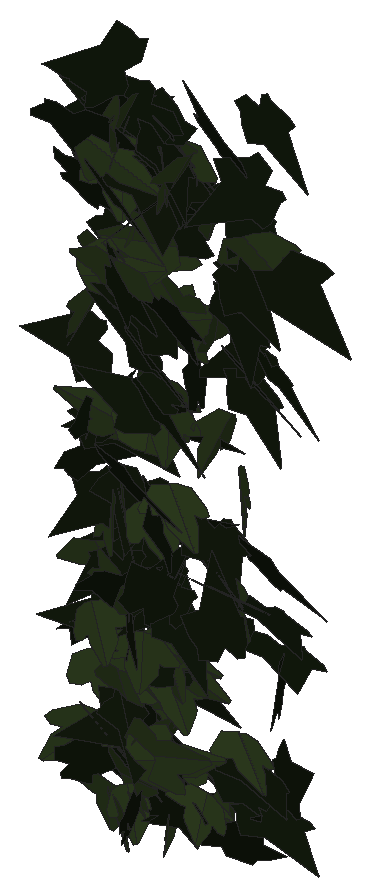
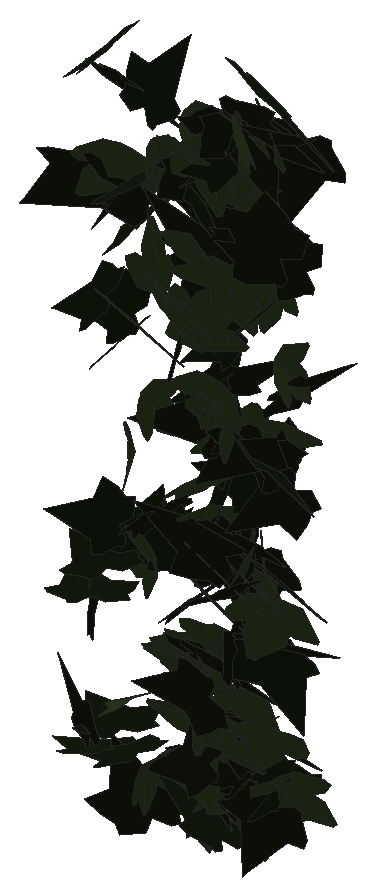
# SketchUp Ruby script. Lengths in inches.
U = 1.inch
M = Sketchup.active_model
def pt(a) = Geom::Point3d.new(a.map { |v| v * U })
def face(e, loops, mat)
  f = e.add_face(loops[0].map { |a| pt(a) })
  loops[1..].each { |l| e.add_face(l.map { |a| pt(a) }).erase! }
  f.material = f.back_material = mat if mat
  f
end
# faces: each face lists its corners as indices into pts; further lists are holes
def faces(e, pts, list, mat = nil) = list.each { |f| face(e, (f[0].is_a?(Array) ? f : [f]).map { |l| l.map { |i| pts[i] } }, mat) }
# xy, xz, yz: faces in a plane at the given z, y or x. An outline is a flat list of corners, or four numbers for a rectangle; further outlines are holes
def ring(l) = l.size == 4 ? [[l[0], l[1]], [l[2], l[1]], [l[2], l[3]], [l[0], l[3]]] : l.each_slice(2).to_a
def flat(e, list, mat, &to3) = list.each { |f| face(e, (f[0].is_a?(Array) ? f : [f]).map { |l| ring(l).map { |u, v| to3.(u, v) } }, mat) }
def xy(e, z, list, mat = nil) = flat(e, list, mat) { |x, y| [x, y, z] }
def xz(e, y, list, mat = nil) = flat(e, list, mat) { |x, z| [x, y, z] }
def yz(e, x, list, mat = nil) = flat(e, list, mat) { |y, z| [x, y, z] }
def lines(e, pts, list) = list.each { |a, b| e.add_line(pt(pts[a]), pt(pts[b])) }
# prism: a flat outline (further loops are holes) pulled along v
def prism(e, loops, v, mat = nil)
  f = face(e, loops, mat); d = Geom::Vector3d.new(v.map { |x| x * U })
  f.pushpull(f.normal.samedirection?(d) ? d.length : -d.length)
end
def box(e, o, s, mat = nil) = prism(e, [[o, [o[0] + s[0], o[1], o[2]], [o[0] + s[0], o[1] + s[1], o[2]], [o[0], o[1] + s[1], o[2]]]], [0, 0, s[2]], mat)
def at(x, y, z, deg = 0) = Geom::Transformation.translation(pt([x, y, z])) * Geom::Transformation.rotation(ORIGIN, Z_AXIS, deg.degrees)
def axes(o, x, y, z) = Geom::Transformation.new([*x, 0, *y, 0, *z, 0, *pt(o).to_a, 1])
def part(name) = M.definitions.add(name)
# library, detail: a bought-in or finely detailed component or shape, given as its bounding box
def library(name, o, s) = part(name).tap { |d| box(d.entities, o, s) }
def detail(e, o, s) = box(e.add_group.entities, o, s)
def put(e, d, t, mat = nil) = e.add_instance(d, t).tap { |i| i.material = mat if mat }
def group(e, t, mat = nil) = e.add_group.tap { |g| g.transformation = t; g.material = mat if mat }.entities
root = M.entities
M.materials.add("1026 AP 7946 SUNNY SIDE UP").color = [254, 231, 186]
M.materials.add("efeu1").color = [18, 25, 13]
M.materials.add("efeu2").color = [43, 57, 29]
c1 = part("ivyleaf_10")
p = [[0,0.5,-0.03],[-0.0625,2.02,-0.43],[-0.19,2.01,-0.46],[-0.54,1.05,-0.29],[-0.52,0.625,-0.18],[-0.83,0.76,-0.28],
  [-1.16,0.64,-0.33],[-1.15,0.33,-0.24],[-0.77,-0.39,0.02],[-0.3,-0.51,0.16],[0.04,-0.48,0.23],[-0.02,2.01,-0.4375],
  [-0.06,2.01,-0.43],[0.04,-0.49,0.23],[0.67,-0.49,0.14],[1.38,0.36,-0.2],[1.375,0.51,-0.24],[0.81,0.65,-0.19],
  [0.62,0.59,-0.15],[0.6,1.09,-0.28],[0.5,1.23,-0.31]]
faces(c1.entities,p,[[0,1,2,3,4,5,6,7,8,9,10],[11,12,0,13,14,15,16,17,18,19,20]],"efeu2")
c2 = part("ivyleaf_9")
p = [[1.54,2.16,1.25],[1.36,2.04,1.19],[-0.21,0.99,0.68],[-0.71,1.11,0.82],[-0.85,0.86,0.67],[-0.8,0.17,0.21],
  [-0.9,-0.01,0.1],[-0.67,-0.16,-0.02],[-0.08,-0.08,-0.05],[-0.03,-0.6,-0.4],[0.65,-0.88,-0.66],[0.83,-0.6,-0.49],
  [1.29,-0.42,-0.43],[1.8125,-0.07,-0.26],[1.21,0.44,0.15]]
faces(c2.entities,p,[[0,1,2,3,4,5,6,7,8,9,10,11,12,13,14]],"efeu1")
put(root,c1,axes([136.93,211.77,280.29],[0.39864,0.12424,-0.25117],[-0.33198,-0.12413,-0.29122],[-0.27527,0.32962,-0.01252]),"1026 AP 7946 SUNNY SIDE UP")
put(root,c2,axes([136.99,212.09,283.83],[-0.49314,0.07212,-0.05929],[0.07158,-0.05806,-0.32851],[-0.12666,-0.31361,0.04519]),"1026 AP 7946 SUNNY SIDE UP")
put(root,c1,axes([136.78,211.9,286.96],[0.07508,-0.29933,0.20921],[0.07253,-0.19986,-0.3132],[0.56563,0.06536,0.01239]),"1026 AP 7946 SUNNY SIDE UP")
put(root,c2,axes([136.35,212.05,288.71],[0.35382,-0.13634,0.24111],[0.27517,-0.16036,-0.26962],[0.32645,0.28295,-0.03405]),"1026 AP 7946 SUNNY SIDE UP")
put(root,c2,axes([136.94,211.81,286.39],[-0.02593,-0.29744,-0.19945],[0.04866,-0.1926,0.30365],[-0.55447,-0.003,0.03598]),"1026 AP 7946 SUNNY SIDE UP")
put(root,c2,axes([136.97,211.34,290.16],[0.48674,0.14403,-0.18455],[-0.23274,-0.10677,-0.35096],[-0.27784,0.34177,-0.02932]),"1026 AP 7946 SUNNY SIDE UP")
put(root,c2,axes([136.93,211.94,280.03],[0.49241,0.07392,-0.1205],[-0.17277,-0.04476,-0.33127],[-0.13316,0.33143,-0.01579]),"1026 AP 7946 SUNNY SIDE UP")
put(root,c2,axes([136.95,211.55,284.83],[-0.02041,0.07372,-0.35573],[-0.11651,0.3377,0.07903],[0.54348,0.07516,0.00358]),"1026 AP 7946 SUNNY SIDE UP")
put(root,c2,axes([137.24,211.61,282.22],[0.0312,0.33207,-0.12146],[-0.07245,-0.11651,-0.34129],[-0.55033,0.03416,0.03805]),"1026 AP 7946 SUNNY SIDE UP")
put(root,c1,axes([137.03,211.86,283.06],[-0.53499,-0.12644,-0.08536],[0.14347,-0.01126,-0.37157],[0.18874,-0.34983,0.04049]),"1026 AP 7946 SUNNY SIDE UP")
put(root,c1,axes([136.92,211.98,281.19],[0.45961,0.15509,0.09905],[0.14745,0.02614,-0.34011],[-0.24529,0.30632,-0.01886]),"1026 AP 7946 SUNNY SIDE UP")
put(root,c2,axes([137.57,211.58,291],[-0.40272,0.31992,0.15659],[-0.18475,0.09785,-0.42057],[-0.5241,-0.28032,0.02793]),"1026 AP 7946 SUNNY SIDE UP")
put(root,c2,axes([137.04,212.34,287.77],[-0.08885,-0.27068,0.21766],[-0.04299,-0.21146,-0.28578],[0.53971,-0.06141,0.01307]),"1026 AP 7946 SUNNY SIDE UP")
put(root,c2,axes([137.48,211.74,285.4375],[-0.32726,0.25952,0.02281],[-0.07406,-0.01151,-0.33979],[-0.40261,-0.20883,0.04396]),"1026 AP 7946 SUNNY SIDE UP")
put(root,c2,axes([137.08,211.49,285.16],[0.0005,-0.04609,0.36122],[0.3436,0.27604,0.03876],[-0.43773,0.21663,0.03084]),"1026 AP 7946 SUNNY SIDE UP")
put(root,c1,axes([137.28,211.58,288.01],[-0.52163,0.16131,0.0163],[-0.04347,-0.0229,-0.37866],[-0.25099,-0.33128,0.0317]),"1026 AP 7946 SUNNY SIDE UP")
put(root,c2,axes([136.96,211.31,279.91],[0.15307,0.07969,0.30415],[0.42767,0.11804,-0.12471],[-0.2183,0.28713,-0.03105]),"1026 AP 7946 SUNNY SIDE UP")
put(root,c1,axes([137.61,211.49,285.51],[0.14265,0.06466,0.33487],[-0.48667,-0.10294,0.10961],[0.18478,-0.32103,0.03016]),"1026 AP 7946 SUNNY SIDE UP")
put(root,c1,axes([137.62,211.36,290.24],[-0.01233,0.08021,0.39313],[-0.49949,0.21928,-0.05299],[-0.3544,-0.31185,0.061]),"1026 AP 7946 SUNNY SIDE UP")
put(root,c2,axes([137.64,211.68,282.27],[-0.37798,0.00609,0.22191],[-0.3256,-0.09571,-0.23586],[0.09364,-0.30824,0.07564]),"1026 AP 7946 SUNNY SIDE UP")
put(root,c1,axes([137.0625,211.93,283.73],[0.20405,-0.09393,0.31687],[0.34377,-0.21827,-0.16469],[0.37198,0.25325,-0.02162]),"1026 AP 7946 SUNNY SIDE UP")
put(root,c2,axes([136.76,212.14,288.83],[0.2823,-0.08921,0.40928],[0.48788,-0.25204,-0.20397],[0.4158,0.3563,-0.03855]),"1026 AP 7946 SUNNY SIDE UP")
put(root,c1,axes([137.25,212.1,284.03],[-0.07396,0.28083,-0.16562],[0.04185,-0.16017,-0.29428],[-0.50835,-0.05405,-0.00013]),"1026 AP 7946 SUNNY SIDE UP")
put(root,c2,axes([137.52,211.74,283.28],[-0.52581,0.06428,-0.12098],[0.16043,-0.08368,-0.34591],[-0.13707,-0.34453,0.05924]),"1026 AP 7946 SUNNY SIDE UP")
put(root,c1,axes([137.71,211.35,282.95],[-0.20558,0.05575,0.30908],[-0.46464,0.05694,-0.14338],[-0.11777,-0.32198,0.02616]),"1026 AP 7946 SUNNY SIDE UP")
put(root,c1,axes([137.41,212.06,289.93],[-0.07296,0.2067,-0.30985],[-0.07696,-0.30514,-0.20923],[-0.5702,0.01473,0.06789]),"1026 AP 7946 SUNNY SIDE UP")
put(root,c1,axes([137.52,211.5,279.56],[-0.4753,0.04032,0.05069],[-0.08344,-0.03005,-0.3121],[-0.05466,-0.30474,0.03565]),"1026 AP 7946 SUNNY SIDE UP")
put(root,c2,axes([137.04,211.82,280.28],[0.33428,-0.25863,0.16353],[0.14298,-0.13249,-0.34543],[0.4565,0.23088,-0.01155]),"1026 AP 7946 SUNNY SIDE UP")
put(root,c2,axes([137.62,211.78,290.4],[0.10188,0.28319,-0.2249],[-0.04468,-0.21872,-0.30006],[-0.56202,0.06872,-0.01691]),"1026 AP 7946 SUNNY SIDE UP")
put(root,c2,axes([137.88,211.78,290.48],[-0.0149,-0.04687,-0.3811],[-0.41566,-0.25977,0.03939],[-0.41294,0.26317,-0.0259]),"1026 AP 7946 SUNNY SIDE UP")
put(root,c1,axes([137.43,211.22,282.47],[0.17588,0.31826,0.00948],[0.01533,0.00441,-0.34741],[-0.50033,0.11201,-0.00731]),"1026 AP 7946 SUNNY SIDE UP")
put(root,c1,axes([137.7,211.3,288.02],[-0.5876,0.01666,0.09381],[-0.14501,-0.03868,-0.3832],[-0.01093,-0.38266,0.04055]),"1026 AP 7946 SUNNY SIDE UP")
put(root,c1,axes([137.57,211.83,290.39],[0.12966,-0.36137,0.10034],[0.01711,-0.09948,-0.38226],[0.5891,0.08243,-0.01098]),"1026 AP 7946 SUNNY SIDE UP")
put(root,c1,axes([137.67,212,287.94],[-0.11616,-0.31092,0.12575],[-0.03937,-0.12132,-0.32991],[0.52476,-0.07793,0.00309]),"1026 AP 7946 SUNNY SIDE UP")
put(root,c1,axes([137.6,211.64,281.3],[-0.52558,0.10178,-0.02684],[0.02429,-0.04026,-0.35849],[-0.16363,-0.33289,0.03299]),"1026 AP 7946 SUNNY SIDE UP")
put(root,c2,axes([137.55,212.1,284.18],[-0.41017,-0.13512,-0.16325],[0.27891,-0.0133,-0.29061],[0.16981,-0.30453,0.08299]),"1026 AP 7946 SUNNY SIDE UP")
put(root,c2,axes([137.36,211.68,285.5],[-0.0797,-0.14271,-0.3437],[0.18445,0.31147,-0.15418],[0.5387,-0.12776,0.00194]),"1026 AP 7946 SUNNY SIDE UP")
put(root,c2,axes([137.95,211.49,280.83],[-0.48105,0.05626,0.10725],[-0.16986,-0.01715,-0.31857],[-0.07486,-0.3226,0.03369]),"1026 AP 7946 SUNNY SIDE UP")
put(root,c2,axes([138.07,211.73,290.01],[-0.09325,0.09619,0.38084],[-0.57632,0.08915,-0.08407],[-0.16621,-0.36308,0.07785]),"1026 AP 7946 SUNNY SIDE UP")
put(root,c1,axes([137.49,211.66,289.4],[0.52881,0.09615,0.04929],[0.08272,-0.01243,-0.35941],[-0.14678,0.33939,-0.02498]),"1026 AP 7946 SUNNY SIDE UP")
put(root,c1,axes([137.98,211.99,280.94],[0.22627,-0.0863,-0.30651],[-0.43366,0.11255,-0.17067],[0.22023,0.31028,-0.02115]),"1026 AP 7946 SUNNY SIDE UP")
put(root,c1,axes([137.35,211.47,289.72],[-0.30172,-0.09486,-0.29096],[0.46756,-0.0538,-0.19019],[0.0103,-0.33673,0.11017]),"1026 AP 7946 SUNNY SIDE UP")
put(root,c2,axes([137.42,211.79,283.93],[0.06748,-0.0427,-0.33349],[0.46238,-0.13631,0.05793],[-0.22231,-0.29648,0.01925]),"1026 AP 7946 SUNNY SIDE UP")
put(root,c2,axes([137.61,211.97,282],[0.04782,0.13868,0.42312],[-0.20909,-0.38806,0.14314],[0.64754,-0.13555,0.01497]),"1026 AP 7946 SUNNY SIDE UP")
put(root,c2,axes([137.37,211.38,289.33],[0.45675,-0.28252,0.02223],[-0.00415,-0.03588,-0.4167],[0.44572,0.28919,-0.02665]),"1026 AP 7946 SUNNY SIDE UP")
put(root,c1,axes([137.68,211.32,279.52],[-0.28001,0.24647,-0.06538],[0.04102,-0.06108,-0.31326],[-0.39864,-0.17941,0.01369]),"1026 AP 7946 SUNNY SIDE UP")
put(root,c1,axes([137.36,211.38,287.79],[0.27127,-0.05329,-0.34809],[0.53275,-0.0229,0.18197],[-0.07044,-0.37842,0.03574]),"1026 AP 7946 SUNNY SIDE UP")
put(root,c1,axes([137.7,211.86,290.13],[-0.43098,-0.1805,-0.13712],[0.26228,-0.02579,-0.32044],[0.23429,-0.30316,0.10649]),"1026 AP 7946 SUNNY SIDE UP")
put(root,c1,axes([138.21,211.63,288.44],[0.20931,-0.06662,-0.35581],[-0.51003,0.11855,-0.15182],[0.21244,0.35027,-0.01393]),"1026 AP 7946 SUNNY SIDE UP")
put(root,c2,axes([137.93,211.17,283.27],[0.24956,0.32164,-0.10605],[-0.05102,-0.10072,-0.36977],[-0.52945,0.16131,-0.01436]),"1026 AP 7946 SUNNY SIDE UP")
put(root,c1,axes([138.09,212.03,289.86],[-0.54056,0.04704,0.1359],[-0.21351,-0.02918,-0.35471],[-0.05232,-0.36697,0.04344]),"1026 AP 7946 SUNNY SIDE UP")
put(root,c2,axes([137.8,211.16,288.08],[0.38523,-0.19837,-0.28642],[-0.33456,0.17723,-0.3237],[0.41825,0.32448,0.00488]),"1026 AP 7946 SUNNY SIDE UP")
put(root,c2,axes([138.03,211.64,286.83],[0.03186,-0.3768,0.00791],[0.01782,0.01044,0.38861],[-0.59242,-0.01995,0.01212]),"1026 AP 7946 SUNNY SIDE UP")
put(root,c2,axes([137.86,212.09,283.14],[-0.23185,-0.28732,0.11258],[-0.01615,-0.11832,-0.33051],[0.48402,-0.14158,0.0429]),"1026 AP 7946 SUNNY SIDE UP")
put(root,c2,axes([137.58,211.66,282.66],[0.01739,-0.1062,-0.42378],[0.61113,-0.16223,0.05304],[-0.2675,-0.37752,0.09363]),"1026 AP 7946 SUNNY SIDE UP")
put(root,c2,axes([138.32,211.87,281.91],[-0.3792,0.12599,0.16898],[-0.24642,0.05144,-0.27899],[-0.21087,-0.28668,0.02215]),"1026 AP 7946 SUNNY SIDE UP")
put(root,c2,axes([138.08,211.86,287.07],[0.03316,-0.36637,-0.07033],[0.00736,-0.06603,0.37767],[-0.58537,-0.02159,0.00077]),"1026 AP 7946 SUNNY SIDE UP")
put(root,c1,axes([137.85,211.45,279.63],[0.19775,0.28098,-0.01252],[0.01181,-0.01841,-0.31689],[-0.44218,0.12517,-0.01407]),"1026 AP 7946 SUNNY SIDE UP")
put(root,c1,axes([137.66,211.59,279.8],[-0.25211,-0.00318,0.30787],[0.44287,-0.11509,0.15373],[0.15725,0.31903,0.06063]),"1026 AP 7946 SUNNY SIDE UP")
put(root,c2,axes([137.86,211.72,280.77],[-0.13229,-0.32043,0.09554],[0.01874,-0.10032,-0.33991],[0.525,-0.07716,0.03621]),"1026 AP 7946 SUNNY SIDE UP")
put(root,c2,axes([137.57,211.48,284.69],[0.32168,-0.19696,0.21194],[0.21293,-0.15713,-0.29303],[0.39542,0.24484,-0.01462]),"1026 AP 7946 SUNNY SIDE UP")
put(root,c2,axes([138.22,211.93,283.5],[-0.46967,0.1199,-0.0451],[0.04815,-0.04261,-0.33058],[-0.19522,-0.29897,0.02697]),"1026 AP 7946 SUNNY SIDE UP")
put(root,c1,axes([138.25,212.03,287.18],[-0.54951,0.01534,-0.17674],[-0.26618,0.04213,0.35919],[0.05075,0.38706,-0.0298]),"1026 AP 7946 SUNNY SIDE UP")
put(root,c2,axes([138.31,211.4,285.92],[-0.10603,0.10099,0.33425],[-0.49992,-0.13404,-0.02592],[0.18614,-0.30245,0.12078]),"1026 AP 7946 SUNNY SIDE UP")
put(root,c1,axes([137.83,212,285.75],[-0.25398,0.11138,-0.28256],[0.23753,-0.2385,-0.19237],[-0.40138,-0.21162,0.06495]),"1026 AP 7946 SUNNY SIDE UP")
put(root,c1,axes([138,211.58,285.34],[0.24112,0.299,-0.17953],[0.08725,0.16877,0.34624],[0.5385,-0.16122,0.02429]),"1026 AP 7946 SUNNY SIDE UP")
put(root,c2,axes([138.05,211.12,279.37],[0.01102,0.03272,0.33814],[0.20251,0.30178,-0.03208],[-0.47719,0.12882,-0.0058]),"1026 AP 7946 SUNNY SIDE UP")
put(root,c2,axes([137.69,212.06,290.05],[0.4629,-0.19329,0.09361],[0.08745,-0.08194,-0.36131],[0.32502,0.29734,-0.03611]),"1026 AP 7946 SUNNY SIDE UP")
put(root,c2,axes([137.71,211.76,280.78],[0.0476,-0.02624,-0.35792],[0.54759,-0.00125,0.03136],[-0.00554,-0.34859,0.02478]),"1026 AP 7946 SUNNY SIDE UP")
put(root,c2,axes([138.52,211.78,281.83],[-0.2706,0.13309,0.25627],[-0.38106,0.07776,-0.21578],[-0.22507,-0.29168,0.05722]),"1026 AP 7946 SUNNY SIDE UP")
put(root,c2,axes([138.29,211.77,289.21],[-0.31059,0.1902,-0.24074],[0.11844,-0.24062,-0.26754],[-0.46009,-0.19034,0.09364]),"1026 AP 7946 SUNNY SIDE UP")
put(root,c1,axes([137.9375,211.88,288.12],[-0.2609,-0.19495,0.27417],[0.21236,0.23299,0.26285],[-0.4748,0.21133,-0.03309]),"1026 AP 7946 SUNNY SIDE UP")
put(root,c2,axes([138.27,211.8125,289.49],[0.14862,0.27194,-0.21457],[-0.06905,-0.20628,-0.29699],[-0.53566,0.10204,-0.02125]),"1026 AP 7946 SUNNY SIDE UP")
put(root,c1,axes([138.02,211.46,282.1],[0.49272,0.03166,0.05162],[0.0831,-0.02936,-0.32272],[-0.04165,0.31594,-0.03328]),"1026 AP 7946 SUNNY SIDE UP")
put(root,c1,axes([138.33,211.68,279.75],[-0.4671,0.13496,-0.11276],[-0.13698,0.07364,0.3352],[0.23729,0.30817,-0.02846]),"1026 AP 7946 SUNNY SIDE UP")
put(root,c1,axes([137.9,211.78,289.24],[0.51442,0.12657,0.1416],[0.22163,0.01256,-0.35934],[-0.1916,0.35435,-0.0355]),"1026 AP 7946 SUNNY SIDE UP")
put(root,c2,axes([137.8125,211.7,280.4],[0.48862,-0.13975,0.07202],[0.0794,-0.05929,-0.34974],[0.2331,0.31312,-0.03182]),"1026 AP 7946 SUNNY SIDE UP")
put(root,c2,axes([138.42,211.79,282.98],[-0.54427,0.13064,-0.09453],[0.11461,-0.06757,-0.37969],[-0.22409,-0.35186,0.0354]),"1026 AP 7946 SUNNY SIDE UP")
put(root,c1,axes([138.12,211.8,286.05],[-0.50622,0.09653,-0.11446],[0.15406,-0.06061,-0.34537],[-0.17358,-0.33532,0.02728]),"1026 AP 7946 SUNNY SIDE UP")
put(root,c1,axes([138.27,211.71,280.78],[-0.06162,-0.34843,0.01596],[0.00282,-0.01778,-0.3613],[0.54855,-0.03905,0.00365]),"1026 AP 7946 SUNNY SIDE UP")
put(root,c1,axes([138.07,211.62,284.11],[0.2288,0.31656,0.07793],[0.07518,0.05918,-0.35808],[-0.50557,0.15206,-0.01798]),"1026 AP 7946 SUNNY SIDE UP")
put(root,c2,axes([137.82,212,283.73],[0.38918,0.15023,-0.1758],[0.20617,0.11328,0.29784],[0.29328,-0.27899,0.0239]),"1026 AP 7946 SUNNY SIDE UP")
put(root,c2,axes([137.96,211.46,286.9],[0.4153,-0.23003,-0.01377],[-0.03277,-0.00559,-0.36039],[0.36071,0.26434,-0.01688]),"1026 AP 7946 SUNNY SIDE UP")
put(root,c2,axes([138.14,211.76,289.54],[-0.37671,-0.22839,-0.19083],[0.2571,0.09313,-0.33798],[0.38276,-0.28733,0.03922]),"1026 AP 7946 SUNNY SIDE UP")
put(root,c2,axes([137.9,211.95,279.29],[0.18214,-0.29811,0.10705],[0.48744,0.12929,0.02646],[-0.09847,0.08862,0.32899]),"1026 AP 7946 SUNNY SIDE UP")
put(root,c1,axes([138.23,211.68,289.4375],[-0.37529,0.26142,0.14992],[0.18781,-0.08537,0.363],[0.43011,0.26538,-0.0277]),"1026 AP 7946 SUNNY SIDE UP")
put(root,c2,axes([138.04,212.01,288.39],[-0.19085,0.1032,0.31474],[0.42594,-0.14333,0.16022],[0.27349,0.29524,-0.02989]),"1026 AP 7946 SUNNY SIDE UP")
put(root,c1,axes([138.38,211.73,279.41],[-0.08232,0.30015,-0.02563],[-0.14322,-0.04148,-0.29797],[-0.45164,-0.04156,0.09916]),"1026 AP 7946 SUNNY SIDE UP")
put(root,c2,axes([138.1,211.93,289.69],[0.05397,-0.33812,0.14326],[0.03661,-0.1393,-0.35082],[0.57485,0.04061,0.00889]),"1026 AP 7946 SUNNY SIDE UP")
put(root,c2,axes([138.02,212.05,280.43],[0.40279,-0.19805,0.10107],[0.10606,-0.07476,-0.33354],[0.33177,0.26434,-0.01607]),"1026 AP 7946 SUNNY SIDE UP")
put(root,c2,axes([137.99,211.74,285.6],[0.40634,-0.01604,0.21777],[0.32979,-0.03017,-0.26656],[0.04952,0.33256,-0.01172]),"1026 AP 7946 SUNNY SIDE UP")
put(root,c2,axes([138.32,211.58,283.96],[-0.10613,-0.02388,0.41954],[-0.08522,-0.40874,-0.03633],[0.63599,-0.05876,0.06514]),"1026 AP 7946 SUNNY SIDE UP")
put(root,c2,axes([138.02,212.07,281.48],[0.10649,-0.01567,-0.34843],[0.50877,0.10427,0.0624],[0.15631,-0.3287,0.03428]),"1026 AP 7946 SUNNY SIDE UP")
put(root,c1,axes([138.29,212,289.72],[0.57583,-0.08475,0.10851],[0.14917,-0.05751,-0.38605],[0.15227,0.37683,-0.03215]),"1026 AP 7946 SUNNY SIDE UP")
put(root,c1,axes([138.29,211.84,281.73],[-0.18868,0.03374,-0.31332],[0.20076,-0.29157,-0.08687],[-0.4376,-0.14831,0.09524]),"1026 AP 7946 SUNNY SIDE UP")
put(root,c1,axes([138.32,211.69,285.8],[0.52327,-0.0806,0.10558],[0.141,-0.06415,-0.35077],[0.14961,0.34239,-0.03868]),"1026 AP 7946 SUNNY SIDE UP")
put(root,c2,axes([138.25,211.72,289.99],[0.08627,-0.34522,0.09461],[0.02919,-0.09202,-0.36062],[0.56175,0.0578,0.00421]),"1026 AP 7946 SUNNY SIDE UP")
put(root,c2,axes([138.18,211.48,286.1],[0.36648,-0.29093,0.01799],[-0.00291,-0.02595,-0.38375],[0.45843,0.23241,-0.01682]),"1026 AP 7946 SUNNY SIDE UP")
put(root,c2,axes([138.76,211.42,279.93],[0.18595,-0.00712,-0.34267],[-0.51563,-0.06185,-0.11912],[-0.08796,0.34752,-0.02612]),"1026 AP 7946 SUNNY SIDE UP")
put(root,c2,axes([138.41,211.08,283.03],[-0.11407,-0.02932,0.38547],[0.3977,0.27797,0.07455],[-0.43637,0.261,-0.03282]),"1026 AP 7946 SUNNY SIDE UP")
put(root,c1,axes([138.17,211.69,282.05],[-0.17709,-0.0173,-0.32255],[0.49267,-0.0167,-0.11529],[-0.01554,-0.33222,0.02063]),"1026 AP 7946 SUNNY SIDE UP")
put(root,c1,axes([138.33,211.7,281.48],[0.43326,0.09107,0.12963],[0.20047,0.01193,-0.29766],[-0.13836,0.30246,-0.02536]),"1026 AP 7946 SUNNY SIDE UP")
put(root,c2,axes([138.47,211.37,287.7],[0.50838,-0.04845,-0.1445],[-0.22448,-0.01223,-0.33539],[0.06216,0.35211,-0.02943]),"1026 AP 7946 SUNNY SIDE UP")
put(root,c1,axes([138.71,211.49,289.92],[0.04285,-0.3592,0.10493],[0.00367,-0.10401,-0.37167],[0.58795,0.02683,-0.00533]),"1026 AP 7946 SUNNY SIDE UP")
put(root,c1,axes([138.46,211.66,284.49],[-0.24768,-0.2937,0.03735],[0.33942,-0.14328,-0.2203],[0.31877,-0.07563,0.26359]),"1026 AP 7946 SUNNY SIDE UP")
put(root,c1,axes([138.26,212.03,287.07],[0.26977,-0.15158,-0.32575],[0.4291,-0.16182,0.23214],[-0.3443,-0.32045,0.03408]),"1026 AP 7946 SUNNY SIDE UP")
put(root,c1,axes([138.32,211.74,279.87],[-0.18682,-0.05004,-0.3372],[0.51673,-0.05803,-0.11418],[-0.06016,-0.34307,0.06639]),"1026 AP 7946 SUNNY SIDE UP")
put(root,c1,axes([138.35,211.79,281.79],[-0.17893,-0.02049,-0.3478],[0.49356,-0.13876,-0.10116],[-0.19761,-0.32802,0.06225]),"1026 AP 7946 SUNNY SIDE UP")
put(root,c1,axes([138.36,211.24,280.52],[-0.30723,0.0151,0.35813],[0.54479,0.04427,0.19894],[-0.04915,0.39624,-0.03353]),"1026 AP 7946 SUNNY SIDE UP")
put(root,c2,axes([138.54,211.66,282.66],[0.10145,-0.34726,-0.04131],[-0.01482,0.03703,-0.36364],[0.54911,0.06516,-0.00218]),"1026 AP 7946 SUNNY SIDE UP")
put(root,c1,axes([138.32,211.27,280.48],[0.15932,-0.01386,-0.38754],[0.58349,0.06864,0.10079],[0.09869,-0.38342,0.02973]),"1026 AP 7946 SUNNY SIDE UP")
put(root,c2,axes([138.87,211.65,286.29],[-0.04495,-0.18981,0.3323],[0.13344,0.31289,0.1986],[-0.57467,0.08751,0.02012]),"1026 AP 7946 SUNNY SIDE UP")
put(root,c2,axes([138.65,211.98,283.52],[0.18263,-0.20114,0.25994],[0.17282,-0.22876,-0.24024],[0.47854,0.15938,-0.01245]),"1026 AP 7946 SUNNY SIDE UP")
put(root,c1,axes([139.03,212.01,285.6875],[-0.02916,-0.29546,0.23017],[0.09021,-0.22496,-0.30063],[0.57705,0.02024,0.05863]),"1026 AP 7946 SUNNY SIDE UP")
put(root,c1,axes([139.13,211.71,289.42],[-0.00963,-0.36098,-0.05735],[0.01817,0.0534,-0.37146],[0.57354,-0.00775,0.01081]),"1026 AP 7946 SUNNY SIDE UP")
put(root,c2,axes([138.95,211.96,283.99],[0.02737,-0.34251,-0.07529],[-0.02406,0.07041,-0.3527],[0.54953,0.02014,-0.01169]),"1026 AP 7946 SUNNY SIDE UP")
put(root,c1,axes([139.125,212.01,279.82],[-0.01451,-0.31446,0.05949],[0.14877,-0.05958,-0.30943],[0.48075,0.00895,0.09755]),"1026 AP 7946 SUNNY SIDE UP")
put(root,c2,axes([139.3,211.77,290.16],[0.2811,-0.30262,0.20963],[-0.12491,0.19082,0.36231],[-0.56118,-0.19405,0.02436]),"1026 AP 7946 SUNNY SIDE UP")
put(root,c1,axes([139.13,211.48,279.95],[-0.2951,-0.1544,0.20176],[0.20994,-0.26983,-0.08854],[0.3325,0.03334,0.23497]),"1026 AP 7946 SUNNY SIDE UP")
put(root,c1,axes([139.29,211.62,287.41],[-0.04259,-0.35435,-0.11792],[-0.02525,-0.11153,0.36538],[-0.58402,0.03066,-0.0072]),"1026 AP 7946 SUNNY SIDE UP")
put(root,c2,axes([139.66,212.09,287.06],[-0.48887,0.14445,0.00484],[-0.02583,-0.0262,-0.35191],[-0.22575,-0.30983,0.02979]),"1026 AP 7946 SUNNY SIDE UP")
put(root,c2,axes([139.31,212.34,289.03],[-0.18945,-0.25835,0.21616],[-0.00337,-0.22403,-0.28477],[0.52477,-0.09471,0.07621]),"1026 AP 7946 SUNNY SIDE UP")
put(root,c1,axes([139.17,211.94,283.17],[-0.23362,0.14311,-0.29721],[0.25001,-0.24471,-0.21026],[-0.44168,-0.21422,0.03819]),"1026 AP 7946 SUNNY SIDE UP")
put(root,c2,axes([139.18,211.86,279.14],[0.52483,0.09235,0.03683],[-0.06688,0.02221,0.35532],[0.1403,-0.3349,0.0316]),"1026 AP 7946 SUNNY SIDE UP")
put(root,c1,axes([139.33,212.1,284.85],[-0.1488,0.21949,-0.27097],[0.08901,-0.26041,-0.24521],[-0.53279,-0.10481,0.03471]),"1026 AP 7946 SUNNY SIDE UP")
put(root,c2,axes([139.45,211.78,283.18],[-0.39861,-0.13083,0.16384],[0.22588,-0.29347,-0.01448],[0.23329,0.06059,0.29397]),"1026 AP 7946 SUNNY SIDE UP")
put(root,c2,axes([139.73,211.18,282.85],[-0.27589,-0.22895,0.2865],[0.22867,0.23956,0.29771],[-0.51992,0.22685,-0.02108]),"1026 AP 7946 SUNNY SIDE UP")
put(root,c2,axes([139.28,212.05,280.15],[0.1779,-0.2994,-0.01337],[0.18673,0.05588,-0.30063],[0.43252,0.09902,0.13528]),"1026 AP 7946 SUNNY SIDE UP")
put(root,c1,axes([139.49,211.89,280.82],[-0.21965,-0.26764,0.11487],[0.37426,-0.17734,-0.1306],[0.26195,0.02895,0.28292]),"1026 AP 7946 SUNNY SIDE UP")
put(root,c2,axes([139.53,212.01,286.5],[0.15436,-0.3456,-0.03278],[-0.0394,0.02389,-0.36954],[0.54402,0.09979,-0.01746]),"1026 AP 7946 SUNNY SIDE UP")
put(root,c2,axes([139.58,212,280.42],[-0.04205,-0.30657,0.12016],[0.30546,-0.11055,-0.25036],[0.41679,0.05009,0.19561]),"1026 AP 7946 SUNNY SIDE UP")
put(root,c2,axes([139.52,211.82,286.84],[0.32732,-0.22671,0.15939],[0.14841,-0.12493,-0.31751],[0.40648,0.22818,-0.01243]),"1026 AP 7946 SUNNY SIDE UP")
put(root,c2,axes([139.72,211.53,287.96],[0.06669,-0.34581,0.12862],[-0.00291,-0.12785,-0.35927],[0.57915,0.03918,-0.01662]),"1026 AP 7946 SUNNY SIDE UP")
put(root,c2,axes([140.21,211.41,290.15],[-0.56832,0.05965,-0.00673],[0.00182,-0.03501,-0.37592],[-0.09439,-0.3598,0.03328]),"1026 AP 7946 SUNNY SIDE UP")
put(root,c2,axes([139.54,212.14,283.68],[0.35614,-0.18201,0.18984],[0.20766,-0.13102,-0.29962],[0.35169,0.26167,-0.01532]),"1026 AP 7946 SUNNY SIDE UP")
put(root,c2,axes([139.83,211.375,288.62],[0.18848,-0.28773,-0.18105],[-0.11797,0.1573,-0.32009],[0.51548,0.1412,-0.00706]),"1026 AP 7946 SUNNY SIDE UP")
put(root,c2,axes([139.72,212.14,282.95],[-0.01915,-0.30048,0.14592],[0.29079,-0.12539,-0.25531],[0.4353,0.07054,0.17697]),"1026 AP 7946 SUNNY SIDE UP")
put(root,c2,axes([139.79,211.93,290.98],[0.2316,-0.33472,-0.07867],[-0.03393,0.07183,-0.3762],[0.53811,0.14859,0.01014]),"1026 AP 7946 SUNNY SIDE UP")
put(root,c1,axes([139.9,211.61,289.02],[-0.43854,-0.13324,-0.18594],[0.2789,0.04341,-0.31643],[0.21444,-0.32895,0.03129]),"1026 AP 7946 SUNNY SIDE UP")
put(root,c2,axes([139.96,212.16,282.43],[-0.15809,-0.29919,0.0877],[0.30867,-0.13169,-0.23407],[0.38037,-0.01748,0.22639]),"1026 AP 7946 SUNNY SIDE UP")
put(root,c2,axes([139.89,211.96,287.03],[0.32956,-0.2895,0.05789],[0.02875,-0.05807,-0.36802],[0.46331,0.20953,-0.01834]),"1026 AP 7946 SUNNY SIDE UP")
put(root,c2,axes([140.04,212.14,280.25],[-0.01131,0.09631,0.34271],[0.11063,-0.32483,0.09671],[0.53236,0.06955,-0.01282]),"1026 AP 7946 SUNNY SIDE UP")
put(root,c2,axes([139.96,211.87,279.9],[0.05886,-0.31428,-0.02276],[0.27487,0.03774,-0.26961],[0.41192,0.01972,0.18316]),"1026 AP 7946 SUNNY SIDE UP")
put(root,c2,axes([140.15,211.9375,282.15],[-0.0148,-0.09838,-0.33745],[0.43425,-0.19461,0.05099],[-0.31582,-0.26296,0.08592]),"1026 AP 7946 SUNNY SIDE UP")
put(root,c2,axes([140.08,211.71,288.71],[-0.1161,-0.16578,-0.42543],[0.48408,0.28194,-0.17205],[0.50333,-0.30939,0.06734]),"1026 AP 7946 SUNNY SIDE UP")
